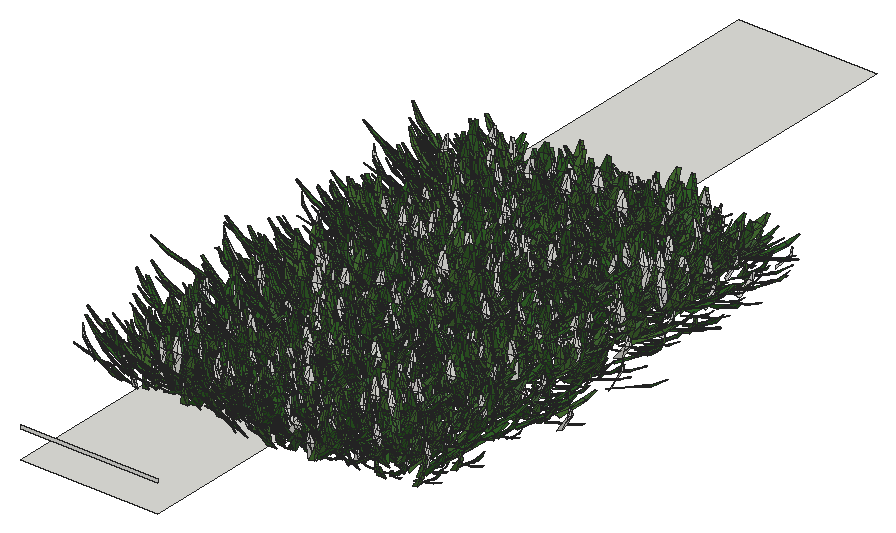
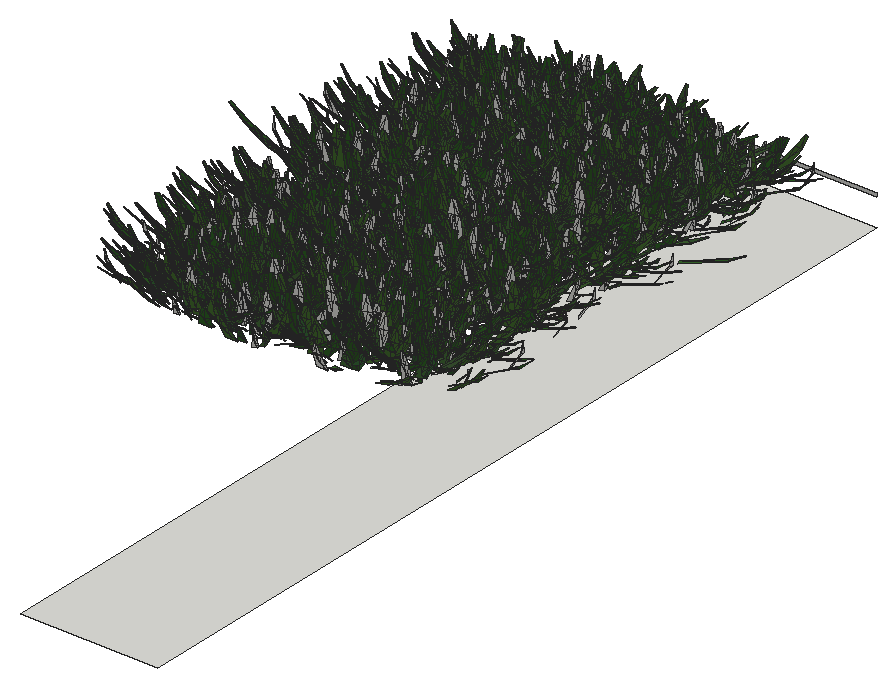
# SketchUp Ruby script. Lengths in inches.
U = 1.inch
M = Sketchup.active_model
def pt(a) = Geom::Point3d.new(a.map { |v| v * U })
def face(e, loops, mat)
  f = e.add_face(loops[0].map { |a| pt(a) })
  loops[1..].each { |l| e.add_face(l.map { |a| pt(a) }).erase! }
  f.material = f.back_material = mat if mat
  f
end
# faces: each face lists its corners as indices into pts; further lists are holes
def faces(e, pts, list, mat = nil) = list.each { |f| face(e, (f[0].is_a?(Array) ? f : [f]).map { |l| l.map { |i| pts[i] } }, mat) }
# xy, xz, yz: faces in a plane at the given z, y or x. An outline is a flat list of corners, or four numbers for a rectangle; further outlines are holes
def ring(l) = l.size == 4 ? [[l[0], l[1]], [l[2], l[1]], [l[2], l[3]], [l[0], l[3]]] : l.each_slice(2).to_a
def flat(e, list, mat, &to3) = list.each { |f| face(e, (f[0].is_a?(Array) ? f : [f]).map { |l| ring(l).map { |u, v| to3.(u, v) } }, mat) }
def xy(e, z, list, mat = nil) = flat(e, list, mat) { |x, y| [x, y, z] }
def xz(e, y, list, mat = nil) = flat(e, list, mat) { |x, z| [x, y, z] }
def yz(e, x, list, mat = nil) = flat(e, list, mat) { |y, z| [x, y, z] }
def lines(e, pts, list) = list.each { |a, b| e.add_line(pt(pts[a]), pt(pts[b])) }
# prism: a flat outline (further loops are holes) pulled along v
def prism(e, loops, v, mat = nil)
  f = face(e, loops, mat); d = Geom::Vector3d.new(v.map { |x| x * U })
  f.pushpull(f.normal.samedirection?(d) ? d.length : -d.length)
end
def box(e, o, s, mat = nil) = prism(e, [[o, [o[0] + s[0], o[1], o[2]], [o[0] + s[0], o[1] + s[1], o[2]], [o[0], o[1] + s[1], o[2]]]], [0, 0, s[2]], mat)
def at(x, y, z, deg = 0) = Geom::Transformation.translation(pt([x, y, z])) * Geom::Transformation.rotation(ORIGIN, Z_AXIS, deg.degrees)
def axes(o, x, y, z) = Geom::Transformation.new([*x, 0, *y, 0, *z, 0, *pt(o).to_a, 1])
def part(name) = M.definitions.add(name)
# library, detail: a bought-in or finely detailed component or shape, given as its bounding box
def library(name, o, s) = part(name).tap { |d| box(d.entities, o, s) }
def detail(e, o, s) = box(e.add_group.entities, o, s)
def put(e, d, t, mat = nil) = e.add_instance(d, t).tap { |i| i.material = mat if mat }
def group(e, t, mat = nil) = e.add_group.tap { |g| g.transformation = t; g.material = mat if mat }.entities
root = M.entities
M.materials.add("Material82").color = [68, 110, 58]
M.materials.add("Material83").color = [48, 90, 38]
M.materials.add("Material84").color = [68, 110, 48]
M.materials.add("Material85").color = [48, 90, 48]
M.materials.add("Material86").color = [58, 110, 58]
M.materials.add("Material87").color = [58, 90, 38]
M.materials.add("Material88").color = [68, 100, 58]
M.materials.add("Material89").color = [48, 100, 38]
c1 = part("grass00")
p = [[-0.6875,0.15,0],[-0.56,0.08,5.52],[-0.04,0.03,2.76],[0.48,-0.02,0],[0.35,-0.02,5.52],[-0.1,-0.14,5.52],
  [-0.12,0.65,8.37],[-0.42,0.65,8.37]]
faces(c1.entities,p,[[0,1,2,3],[3,2,4],[1,5,2],[5,4,2],[1,6,5],[4,5,6],[7,6,1]])
c2 = part("Group16\#1")
put(c2.entities,c1,axes([1.44,-0.61,-0.01],[0.05352,0.12609,0],[-0.10704,0.04543,0.07239],[0.06664,-0.02828,0.11628]),"Material85")
put(c2.entities,c1,axes([0.76,-0.15,-0.01],[0.04676,0.24062,0],[-0.23162,0.04501,0.06642],[0.0652,-0.01267,0.23595]),"Material82")
put(c2.entities,c1,axes([0.79,0.01,-0.01],[-0.00606,0.34651,0],[-0.34381,-0.00602,0.0432],[0.04319,0.00076,0.34386]))
put(c2.entities,c1,axes([1,0.23,-0.01],[-0.07192,0.31144,0],[-0.28722,-0.06632,0.1236],[0.12043,0.02781,0.29478]),"Material84")
put(c2.entities,c1,axes([1.66,0.77,-0.01],[-0.13828,0.29651,0],[-0.21551,-0.1005,0.22471],[0.20365,0.09498,0.23779]),"Material89")
put(c2.entities,c1,axes([0.6875,0.52,-0.01],[-0.18126,0.24051,0],[-0.22746,-0.17142,0.09788],[0.07817,0.05891,0.28481]),"Material84")
put(c2.entities,c1,axes([0.68,0.78,-0.01],[-0.215,0.18688,0],[-0.12385,-0.14248,0.21334],[0.13995,0.16101,0.18878]),"Material82")
put(c2.entities,c1,axes([0.56,1,-0.01],[-0.13756,0.07624,0],[-0.06159,-0.11112,0.0927],[0.04494,0.08108,0.12705]),"Material84")
put(c2.entities,c1,axes([0.2,0.64,-0.01],[-0.23729,0.07254,0],[-0.05711,-0.18681,0.153],[0.04473,0.14632,0.19535]),"Material89")
put(c2.entities,c1,axes([0.0625,0.72,-0.01],[-0.28874,0.02525,0],[-0.02179,-0.24916,0.14647],[0.01276,0.14591,0.25012]),"Material82")
put(c2.entities,c1,axes([-0.08,0.62,-0.01],[-0.34089,-0.04187,0],[0.03255,-0.26504,0.216],[-0.02633,0.21439,0.26703]),"Material89")
put(c2.entities,c1,axes([-0.34,0.98,-0.01],[-0.14314,-0.0493,0],[0.04397,-0.12769,0.06843],[-0.02228,0.0647,0.13505]),"Material89")
put(c2.entities,c1,axes([-0.87,1.45,-0.01],[-0.23488,-0.14114,0],[0.13761,-0.22901,0.06087],[-0.03135,0.05217,0.26717]))
put(c2.entities,c1,axes([-0.72,0.77,-0.01],[-0.14208,-0.13251,0],[0.07209,-0.0773,0.16301],[-0.11118,0.11922,0.1057]),"Material89")
put(c2.entities,c1,axes([-0.62,0.43,-0.01],[-0.14845,-0.21203,0],[0.18654,-0.13061,0.12304],[-0.10079,0.07057,0.22772]),"Material82")
put(c2.entities,c1,axes([-0.68,0.29,-0.01],[-0.13639,-0.32136,0],[0.31723,-0.13464,0.05579],[-0.05136,0.0218,0.34462]),"Material83")
put(c2.entities,c1,axes([-0.64,0.125,-0.01],[-0.0458,-0.23569,0],[0.22124,-0.043,0.08276],[-0.08124,0.01579,0.22538]),"Material86")
put(c2.entities,c1,axes([-1.6,-0.03,-0.01],[0.00576,-0.32897,0],[0.27526,0.00482,0.18018],[-0.18015,-0.00315,0.2753]),"Material84")
put(c2.entities,c1,axes([-1.36,-0.31,-0.01],[0.05718,-0.24765,0],[0.18172,0.04196,0.17267],[-0.16825,-0.03885,0.1865]),"Material89")
put(c2.entities,c1,axes([-1.54,-0.72,-0.01],[0.06537,-0.14017,0],[0.13555,0.06321,0.03939],[-0.0357,-0.01665,0.14956]))
put(c2.entities,c1,axes([-1.19,-0.9,-0.01],[0.09597,-0.12735,0],[0.11214,0.08451,0.07557],[-0.06035,-0.04548,0.14042]),"Material88")
put(c2.entities,c1,axes([-0.47,-0.54,-0.01],[0.11588,-0.10072,0],[0.0618,0.0711,0.12124],[-0.07953,-0.0915,0.0942]))
put(c2.entities,c1,axes([-0.47,-0.84,-0.01],[0.11927,-0.0661,0],[0.06603,0.11913,0.00646],[-0.00313,-0.00565,0.13621]),"Material84")
put(c2.entities,c1,axes([-0.38,-1.24,-0.01],[0.28037,-0.08571,0],[0.0618,0.20215,0.20315],[-0.05939,-0.19428,0.21139]),"Material88")
put(c2.entities,c1,axes([-0.06,-0.66,-0.01],[0.22719,-0.01987,0],[0.01247,0.14255,0.17758],[-0.01547,-0.17691,0.1431]),"Material87")
put(c2.entities,c1,axes([0.11,-0.89,-0.01],[0.14882,0.01828,0],[-0.01058,0.08611,0.12229],[0.01491,-0.12138,0.08676]),"Material85")
put(c2.entities,c1,axes([0.25,-0.72,-0.01],[0.20481,0.07053,0],[-0.06206,0.18022,0.10291],[0.03351,-0.0973,0.1906]),"Material85")
put(c2.entities,c1,axes([0.85,-1.42,-0.01],[0.16481,0.09904,0],[-0.09472,0.15762,0.05616],[0.02893,-0.04814,0.18389]),"Material84")
put(c2.entities,c1,axes([1.01,-1.09,-0.01],[0.21858,0.20385,0],[-0.17495,0.1876,0.15339],[0.10462,-0.11218,0.25652]),"Material89")
put(c2.entities,c1,axes([1.01,-0.71,-0.01],[0.08733,0.12473,0],[-0.06445,0.04512,0.13037],[0.1068,-0.07477,0.07867]),"Material85")
c3 = part("Group15\#1")
put(c3.entities,c2,at(0,0,0))
c4 = part("3darcstudiotree_grass00\#1")
put(c4.entities,c3,at(0,0,0))
xy(root,-42.1875,[[1657.41,273.41,1674.99,387.84]])
xz(root,273.41,[[1657.41,-38.61,1674.99,-38.1875]])
put(root,c4,axes([1666.34,286.12,-34.17],[1.73893,-1.7168,0],[3.5493,0.55914,-0.05078],[0.28442,0.04481,1.72798]))
put(root,c4,axes([1665.54,283.25,-34.17],[1.27117,1.29221,0],[-3.51403,0.53763,-0.02781],[-0.14445,0.0221,1.57422]))
put(root,c4,axes([1667.02,309.98,-34.17],[1.49045,-1.29572,0],[4.01852,0.71892,-0.00454],[0.01627,0.00291,1.30224]))
put(root,c4,axes([1665.8,293.86,-34.17],[3.40006,0.04588,0],[-0.15479,1.78412,-0.02332],[-0.00425,0.049,1.80921]))
put(root,c4,axes([1665.56,329.67,-34.17],[1.48796,1.33204,0],[-3.50735,0.60935,-0.02705],[-0.13278,0.02307,1.54111]))
put(root,c4,axes([1667.26,332.66,-34.17],[-3.4737,0.48099,0],[-1.22806,-1.37939,-0.01418],[-0.03068,-0.03446,1.8149]))
put(root,c4,axes([1666.03,322.07,-34.17],[1.0762,1.29593,0],[-3.71861,0.48029,-0.00037],[-0.00166,0.00021,1.37352]))
put(root,c4,axes([1667.74,303,-34.17],[-4.57816,0.34958,0],[-0.88534,-1.8033,-0.01839],[-0.0151,-0.03075,1.50803]))
put(root,c4,axes([1667.97,291.15,-34.17],[-1.62742,-1.17488,0],[3.69115,-0.79521,-0.05959],[0.21649,-0.04664,1.30502]))
put(root,c4,axes([1667.19,320.27,-34.17],[1.77469,-1.16148,0],[2.86416,0.68064,-0.04784],[0.28474,0.06767,1.7418]))
put(root,c4,axes([1668.11,326.4375,-34.17],[-0.38907,-1.30448,0],[3.64191,-0.16894,-0.01277],[0.06378,-0.00296,1.38207]))
put(root,c4,axes([1666.65,318.48,-34.17],[0.22262,1.70783,0],[-4.21483,0.08545,-0.0387],[-0.20922,0.00424,1.71236]))
put(root,c4,axes([1666.48,306.94,-34.17],[1.40686,1.47706,0],[-4.38712,0.6499,-0.05425],[-0.24934,0.03694,1.72469]))
put(root,c4,axes([1666.91,335.93,-34.17],[3.74197,-0.40965,0],[1.02528,1.45661,-0.05393],[0.09104,0.12934,1.81331]))
put(root,c4,axes([1667.43,289.47,-34.17],[-1.63246,1.63511,0],[-3.4831,-0.54085,-0.00571],[-0.03452,-0.00536,1.8245]))
put(root,c4,axes([1667.63,298.92,-34.17],[-0.95146,1.7451,0],[-3.70497,-0.31417,-0.03186],[-0.21482,-0.01822,1.95913]))
put(root,c4,axes([1668.68,331.43,-34.17],[3.26505,-0.4107,0],[1.3901,1.71877,-0.05774],[0.0978,0.12093,1.91123]))
put(root,c4,axes([1668.51,314.42,-34.17],[2.80643,0.90661,0],[-2.10951,1.0156,-0.00694],[-0.02809,0.01352,1.5947]))
put(root,c4,axes([1668.74,296.95,-34.17],[4.57178,0.1006,0],[-0.19659,1.38952,-0.03032],[-0.00983,0.06951,1.54015]))
put(root,c4,axes([1670.42,331.34,-34.17],[-3.18088,-0.40858,0],[1.35408,-1.63957,-0.00123],[0.00227,-0.00275,1.95221]))
put(root,c4,axes([1671.25,296.25,-34.17],[-2.17426,-1.31341,0],[3.93463,-1.01304,-0.04707],[0.15585,-0.04013,1.39282]))
put(root,c4,axes([1670.89,287.45,-34.17],[-3.35474,0.10257,0],[-0.29043,-1.4774,-0.03359],[-0.01806,-0.09187,1.95875]))
put(root,c4,axes([1670.53,318.16,-34.17],[3.26089,-0.9276,0],[2.41726,1.32164,-0.00659],[0.02436,0.01332,1.95827]))
put(root,c4,axes([1670.33,283.82,-34.17],[3.92346,-0.38379,0],[1.02863,1.63546,-0.04456],[0.04806,0.07641,1.43455]))
put(root,c4,axes([1672,313.41,-34.17],[-3.24318,-0.61658,0],[1.47082,-1.20323,-0.00927],[0.0316,-0.02585,1.99366]))
put(root,c4,axes([1672.55,293.77,-34.17],[-0.91872,-1.28532,0],[4.49567,-0.49978,-0.01485],[0.07367,-0.00819,1.80381]))
put(root,c4,axes([1671.83,307.1,-34.17],[0.6017,-1.37989,0],[3.88457,0.26344,-0.05034],[0.29768,0.02019,1.77282]))
put(root,c4,axes([1671.1875,285.4,-34.17],[3.93415,-0.89756,0],[1.9948,1.35987,-0.042],[0.11006,0.07503,1.56273]))
put(root,c4,axes([1671.37,335.04,-34.17],[-1.11116,1.30676,0],[-3.31516,-0.43843,-0.03292],[-0.23061,-0.0305,1.93659]))
put(root,c4,axes([1672.71,319.98,-34.17],[-1.52685,-1.32373,0],[3.20025,-0.57411,-0.03768],[0.23061,-0.04137,1.77164]))
put(root,c4,axes([1671.8,325.38,-34.17],[-1.03634,1.43503,0],[-4.07668,-0.45789,-0.05457],[-0.22787,-0.02559,1.37935]))
put(root,c4,axes([1673.05,326.875,-34.17],[-3.57412,-0.0033,0],[0.00935,-1.57631,-0.04252],[0.00057,-0.09613,1.71753]))
put(root,c4,axes([1672.76,323.15,-34.17],[1.46562,-1.72266,0],[4.03529,0.53396,-0.04434],[0.25483,0.03372,1.93394]))
put(root,c4,axes([1671.59,304.17,-34.17],[3.29517,0.70525,0],[-2.24642,1.63243,-0.00178],[-0.00323,0.00235,1.34491]))
put(root,c4,axes([1673.5,291.3,-34.17],[-3.95181,0.01249,0],[-0.03447,-1.69649,-0.00779],[-0.00033,-0.01629,1.71052]))
put(root,c4,axes([1672.0625,332.5625,-34.17],[0.85595,1.34318,0],[-4.39323,0.43542,-0.04255],[-0.19043,0.01887,1.5668]))
put(root,c4,axes([1673.12,298.65,-34.17],[2.65299,-0.97546,0],[3.20943,1.35758,-0.02398],[0.06395,0.02705,1.37951]))
put(root,c4,axes([1672.28,315.24,-34.17],[-0.08871,1.46443,0],[-4.0853,-0.03849,-0.0357],[-0.16722,-0.00158,1.43525]))
put(root,c4,axes([1672.9375,302.09,-34.17],[-1.54224,1.54277,0],[-3.96225,-0.61604,-0.03242],[-0.18554,-0.02885,1.96368]))
put(root,c4,axes([1673.8,289.625,-34.17],[1.45525,-1.36358,0],[3.3603,0.55776,-0.00467],[0.02235,0.00371,1.41828]))
put(root,c4,axes([1673.26,328.28,-34.17],[3.00061,-1.20381,0],[2.59687,1.00673,-0.02297],[0.10061,0.039,1.67632]))
put(root,c4,axes([1673.2,338.31,-34.17],[3.81318,-1.10593,0],[2.582,1.38461,-0.02397],[0.05758,0.03088,1.32443]))
put(root,c4,axes([1674.27,300.13,-34.17],[-4.06047,-0.30244,0],[0.85134,-1.77769,-0.03943],[0.03436,-0.07175,1.61444]))
put(root,c4,axes([1672.76,311.82,-34.17],[4.70379,-0.18713,0],[0.44198,1.72795,-0.01121],[0.00446,0.01743,1.30781]))
put(root,c4,axes([1673.62,309.8,-34.17],[4.53982,0.21063,0],[-0.49544,1.66085,-0.02625],[-0.01899,0.06364,1.96735]))
put(root,c4,axes([1675.79,287.28,-34.17],[-3.49662,-0.83415,0],[2.45665,-1.60161,-0.00291],[0.00652,-0.00425,1.54121]))
put(root,c4,axes([1675.96,296.14,-34.17],[0.98995,-1.43102,0],[4.03348,0.43397,-0.01691],[0.08344,0.00898,1.6028]))
put(root,c4,axes([1676.05,319.87,-34.17],[2.00913,-1.08398,0],[3.65765,1.05439,-0.0361],[0.15471,0.0446,1.80295]))
put(root,c4,axes([1675.89,333.45,-34.17],[-2.26736,0.9467,0],[-3.26135,-1.21483,-0.01576],[-0.0639,-0.0238,1.87507]))
put(root,c4,axes([1676.31,310.1,-34.17],[3.78243,-0.20016,0],[0.50434,1.48226,-0.04419],[0.03105,0.09126,1.50171]))
put(root,c4,axes([1677.36,330.47,-34.17],[-3.45253,0.27622,0],[-0.72182,-1.40321,-0.01756],[-0.02267,-0.04407,1.76676]))
put(root,c4,axes([1676.19,283.46,-34.17],[3.16343,0.45899,0],[-1.51538,1.62437,-0.05896],[-0.12026,0.12891,1.94308]))
put(root,c4,axes([1677.36,335.34,-34.17],[0.78455,-1.57227,0],[3.87046,0.30038,-0.05061],[0.32766,0.02543,1.95081]))
put(root,c4,axes([1677.9,314.09,-34.17],[-4.25587,0.04591,0],[-0.1089,-1.57017,-0.04984],[-0.00682,-0.0984,1.49526]))
put(root,c4,axes([1677.88,315.32,-34.17],[0.66389,-1.49509,0],[4.57403,0.31589,-0.04237],[0.23153,0.01599,1.93074]))
put(root,c4,axes([1677.33,307.87,-34.17],[-2.17136,1.02025,0],[-2.89421,-0.95801,-0.02769],[-0.1122,-0.03714,1.49833]))
put(root,c4,axes([1677.42,300.01,-34.17],[-1.21684,1.60263,0],[-3.24686,-0.38342,-0.04102],[-0.25836,-0.03051,1.67021]))
put(root,c4,axes([1677.96,298.69,-34.17],[-3.24632,0.41503,0],[-1.13877,-1.38534,-0.02033],[-0.04358,-0.05301,1.92362]))
put(root,c4,axes([1677.0625,326.37,-34.17],[3.77678,0.27869,0],[-0.6902,1.45473,-0.00485],[-0.00557,0.01174,1.75633]))
put(root,c4,axes([1676.94,289.48,-34.17],[0.70399,1.48206,0],[-4.34932,0.32132,-0.00799],[-0.0357,0.00264,1.50733]))
put(root,c4,axes([1677.66,303.2,-34.17],[4.36912,-0.54802,0],[1.07763,1.33621,-0.00335],[0.00554,0.00687,1.45436]))
put(root,c4,axes([1678.55,337.63,-34.17],[1.61856,-1.20753,0],[3.98562,0.83088,-0.05061],[0.25894,0.05398,1.95538]))
put(root,c4,axes([1679.33,284.88,-34.17],[-4.39724,-0.41789,0],[0.97106,-1.58919,-0.03666],[0.03598,-0.05889,1.30149]))
put(root,c4,axes([1679.63,291.59,-34.17],[-3.07103,-1.30718,0],[3.25603,-1.18973,-0.02123],[0.06738,-0.02462,1.43939]))
put(root,c4,axes([1678.17,318.12,-34.17],[3.97153,-0.13343,0],[0.30373,1.40602,-0.01096],[0.00672,0.03109,1.93666]))
put(root,c4,axes([1679.47,324.36,-34.17],[0.94741,-1.42267,0],[3.73003,0.38633,-0.03356],[0.18091,0.01874,1.61101]))
put(root,c4,axes([1678.45,294.03,-34.17],[3.9873,-0.15062,0],[0.35569,1.46445,-0.02913],[0.01977,0.08141,1.9903]))
put(root,c4,axes([1679.81,311.43,-34.17],[0.11291,-1.83708,0],[4.52912,0.0433,-0.04883],[0.22915,0.00219,1.59403]))
put(root,c4,axes([1678.15,304.79,-34.17],[1.39223,1.25256,0],[-3.795,0.65605,-0.01361],[-0.06427,0.01111,1.60179]))
put(root,c4,axes([1678.93,322.18,-34.17],[4.35154,-0.63119,0],[1.42423,1.52711,-0.01984],[0.04228,0.04533,1.90869]))
put(root,c4,axes([1679.34,328.61,-34.17],[2.81234,1.34734,0],[-2.81254,0.91306,-0.01155],[-0.05543,0.018,1.69697]))
put(root,c4,axes([1681.53,301.41,-34.17],[-3.18803,-0.40221,0],[1.38309,-1.70502,-0.00535],[0.00805,-0.00992,1.67969]))
put(root,c4,axes([1681.68,309.92,-34.17],[0.12157,-1.62148,0],[4.39568,0.05126,-0.0158],[0.08264,0.00096,1.72451]))
put(root,c4,axes([1681.9375,289.96,-34.17],[0.05707,-1.33182,0],[4.67038,0.03113,-0.02351],[0.10833,0.00072,1.61343]))
put(root,c4,axes([1681.33,297.8125,-34.17],[2.55829,-1.10547,0],[3.21956,1.15881,-0.03913],[0.13719,0.04938,1.55084]))
put(root,c4,axes([1682.01,315.66,-34.17],[-4.65824,0.34825,0],[-0.74927,-1.55877,-0.04366],[-0.04609,-0.09588,1.70895]))
put(root,c4,axes([1682.33,307.59,-34.17],[-4.52964,-0.09494,0],[0.22898,-1.69903,-0.02618],[0.00745,-0.05528,1.73378]))
put(root,c4,axes([1682.67,326.74,-34.17],[-3.60203,-0.72226,0],[1.64221,-1.27378,-0.05096],[0.13667,-0.10601,1.60728]))
put(root,c4,axes([1681.43,325.2,-34.17],[3.44825,-0.26897,0],[0.66516,1.32629,-0.00259],[0.00332,0.00662,1.70099]))
put(root,c4,axes([1681.76,320.69,-34.17],[3.35413,-0.63199,0],[1.61191,1.33051,-0.01719],[0.04506,0.03719,1.70421]))
put(root,c4,axes([1683.05,331.67,-34.17],[-3.59651,-0.44623,0],[1.25179,-1.56915,-0.00258],[0.00335,-0.0042,1.35273]))
put(root,c4,axes([1683.37,291.83,-34.17],[-3.14814,-1.33954,0],[3.08708,-1.12839,-0.01903],[0.08494,-0.03105,1.91973]))
put(root,c4,axes([1682.36,302.16,-34.17],[-2.16052,1.42464,0],[-3.02099,-0.71254,-0.01081],[-0.04852,-0.01144,1.38013]))
put(root,c4,axes([1682.83,335.55,-34.17],[1.98347,-1.087,0],[3.74124,1.06175,-0.05142],[0.23843,0.06767,1.97373]))
put(root,c4,axes([1681.92,305.125,-34.17],[1.97793,1.10174,0],[-3.47293,0.96971,-0.06047],[-0.20758,0.05796,1.34144]))
put(root,c4,axes([1683.66,329.35,-34.17],[-1.19412,-1.34448,0],[3.1862,-0.44013,-0.02961],[0.14836,-0.02049,1.34337]))
put(root,c4,axes([1682.78,296.48,-34.17],[-1.72626,1.58438,0],[-3.31687,-0.56206,-0.02574],[-0.1159,-0.01964,1.32606]))
put(root,c4,axes([1682.78,314.18,-34.17],[2.97087,-0.63768,0],[1.76888,1.28171,-0.04084],[0.13668,0.09904,1.94165]))
put(root,c4,axes([1684.41,318.24,-34.17],[-2.73035,-0.81396,0],[2.55013,-1.33042,-0.03674],[0.11326,-0.05909,1.62045]))
put(root,c4,axes([1684.4,286.92,-34.17],[-4.52935,0.02332,0],[-0.05756,-1.73901,-0.02897],[-0.00164,-0.04958,1.4344]))
put(root,c4,axes([1683.26,332.6875,-34.17],[3.47707,-0.28838,0],[0.88445,1.65855,-0.04208],[0.03591,0.06734,1.3356]))
put(root,c4,axes([1683.17,283.95,-34.17],[3.17869,1.06939,0],[-2.97014,1.37309,-0.05603],[-0.1904,0.08802,1.79617]))
put(root,c4,axes([1684.53,294.24,-34.17],[-2.94959,0.77761,0],[-1.85667,-1.09533,-0.00767],[-0.02785,-0.01643,1.63569]))
put(root,c4,axes([1684.83,323.12,-34.17],[1.55533,-1.52655,0],[4.26431,0.67573,-0.03894],[0.20513,0.0325,1.95573]))
put(root,c4,axes([1684.68,312.12,-34.17],[2.20471,-1.56419,0],[3.09714,0.67895,-0.02727],[0.12975,0.02844,1.44583]))
put(root,c4,axes([1685.1,339.89,-34.17],[0.44293,-1.56057,0],[3.90028,0.17217,-0.04376],[0.2246,0.00991,1.51939]))
put(root,c4,axes([1684.13,285.08,-34.17],[4.17705,-0.03481,0],[0.09875,1.84286,-0.00824],[0.00079,0.01483,1.59977]))
put(root,c4,axes([1684.7,337.99,-34.17],[-2.26608,1.33318,0],[-3.11704,-0.82402,-0.02214],[-0.10686,-0.02825,1.63462]))
put(root,c4,axes([1684.54,281.59,-34.17],[3.74746,0.48768,0],[-1.05117,1.25627,-0.0401],[-0.08448,0.10096,1.69032]))
put(root,c4,axes([1686.92,318.45,-34.17],[-4.55367,0.27818,0],[-0.67765,-1.72528,-0.03016],[-0.02264,-0.05764,1.62739]))
put(root,c4,axes([1687.875,305.5625,-34.17],[-1.63823,-1.36099,0],[3.49292,-0.65391,-0.00409],[0.01763,-0.0033,1.3842]))
put(root,c4,axes([1687.32,282.83,-34.17],[-3.4101,0.33219,0],[-0.86784,-1.38556,-0.03348],[-0.045,-0.07185,1.52035]))
put(root,c4,axes([1687.74,306.59,-34.17],[2.36777,-1.25491,0],[3.70344,1.08678,-0.00846],[0.02737,0.00803,1.39582]))
put(root,c4,axes([1688.55,330.67,-34.17],[-4.42879,-0.33071,0],[0.76141,-1.58586,-0.02653],[0.02727,-0.05679,1.69452]))
put(root,c4,axes([1688.54,299,-34.17],[-3.60435,-0.22712,0],[0.60496,-1.49319,-0.01241],[0.00897,-0.02215,1.31731]))
put(root,c4,axes([1687.44,311.36,-34.17],[3.96894,-0.58875,0],[1.33194,1.3965,-0.01237],[0.02838,0.02976,1.84855]))
put(root,c4,axes([1688.94,286.82,-34.17],[-3.95806,-0.26007,0],[0.56997,-1.34913,-0.01531],[0.01744,-0.04128,1.80136]))
put(root,c4,axes([1688.8,291.09,-34.17],[0.93986,-1.61608,0],[3.43783,0.31095,-0.013],[0.09422,0.00852,1.96601]))
put(root,c4,axes([1689.21,294.27,-34.17],[-0.9687,-1.6973,0],[3.99206,-0.35436,-0.03143],[0.1527,-0.01355,1.52743]))
put(root,c4,axes([1689.51,316.53,-34.17],[-1.5733,-1.53629,0],[3.8056,-0.60614,-0.01424],[0.06159,-0.00981,1.43479]))
put(root,c4,axes([1689.37,332.76,-34.17],[-3.45853,-0.30921,0],[0.875,-1.52216,-0.03754],[0.05438,-0.09459,1.94323]))
put(root,c4,axes([1689.07,295.6,-34.17],[-0.43954,-1.59759,0],[3.53501,-0.15126,-0.05057],[0.33495,-0.01433,1.77563]))
put(root,c4,axes([1688.06,309.33,-34.17],[3.08639,0.66231,0],[-1.76537,1.27948,-0.04213],[-0.09869,0.07153,1.35679]))
put(root,c4,axes([1689.27,290.28,-34.17],[2.93587,-1.18133,0],[2.75704,1.06566,-0.0131],[0.05816,0.02248,1.79861]))
put(root,c4,axes([1690.12,319.46,-34.17],[-3.47148,-0.32447,0],[1.09042,-1.81447,-0.00987],[0.00954,-0.01587,1.48448]))
put(root,c4,axes([1688.3,302.78,-34.17],[3.59479,1.11581,0],[-2.65109,1.32837,-0.01986],[-0.0739,0.03703,1.93312]))
put(root,c4,axes([1689.12,285.5625,-34.17],[-0.72391,1.71321,0],[-3.27988,-0.21555,-0.00349],[-0.01869,-0.00123,1.35435]))
put(root,c4,axes([1689.125,337.3125,-34.17],[3.93037,0.00712,0],[-0.01552,1.3324,-0.03904],[-0.00131,0.11261,1.85207]))
put(root,c4,axes([1690.13,299.85,-34.17],[1.97331,-1.7001,0],[3.41411,0.61633,-0.04178],[0.21918,0.03957,1.62381]))
put(root,c4,axes([1689.27,313.02,-34.17],[3.30561,0.92504,0],[-2.54174,1.41264,-0.05586],[-0.15004,0.08339,1.52805]))
put(root,c4,axes([1690.21,329.125,-34.17],[3.0975,-0.44176,0],[1.39811,1.52468,-0.04794],[0.07202,0.07854,1.36124]))
put(root,c4,axes([1690.95,327.59,-34.17],[2.99585,-0.78884,0],[2.43675,1.4393,-0.03164],[0.10153,0.05997,1.90074]))
put(root,c4,axes([1690.59,335.03,-34.17],[4.2542,-0.55295,0],[1.2277,1.46904,-0.0158],[0.03318,0.0397,1.97161]))
put(root,c4,axes([1690.24,325.14,-34.17],[1.7248,1.72946,0],[-3.94677,0.61218,-0.01805],[-0.10059,0.0156,1.90362]))
put(root,c4,axes([1690.24,339.14,-34.17],[0.74688,1.42324,0],[-4.33801,0.35406,-0.00233],[-0.01216,0.00099,1.77271]))
put(root,c4,axes([1690.79,321.9375,-34.17],[4.44722,-0.53115,0],[1.26492,1.64719,-0.03542],[0.04521,0.05887,1.44036]))
put(root,c4,axes([1692.55,305.17,-34.17],[-2.92804,-0.86099,0],[2.52273,-1.33432,-0.01853],[0.05328,-0.02818,1.52144]))
put(root,c4,axes([1692.84,316.7,-34.17],[-3.6982,-1.11774,0],[2.6803,-1.37926,-0.01589],[0.04062,-0.0209,1.38765]))
put(root,c4,axes([1692.52,322.29,-34.17],[-4.1478,0.13224,0],[-0.279,-1.36104,-0.02584],[-0.01399,-0.06822,1.74304]))
put(root,c4,axes([1692.41,329.11,-34.17],[2.38875,-0.89777,0],[2.38741,0.98797,-0.03437],[0.15253,0.06312,1.66865]))
put(root,c4,axes([1693.1,333.22,-34.17],[0.38467,-1.72776,0],[3.7527,0.12994,-0.02351],[0.1369,0.00474,1.65028]))
put(root,c4,axes([1693.69,339.19,-34.17],[-0.80049,-1.46058,0],[4.26303,-0.36338,-0.06129],[0.24511,-0.02089,1.3376]))
put(root,c4,axes([1692.5,300.5,-34.17],[3.0128,0.96923,0],[-2.26467,1.09486,-0.0073],[-0.03331,0.01611,1.93831]))
put(root,c4,axes([1694.47,334.76,-34.17],[-4.20928,0.13814,0],[-0.29813,-1.41294,-0.01346],[-0.00713,-0.03379,1.72106]))
put(root,c4,axes([1694.72,287.39,-34.17],[-3.15856,-0.38514,0],[1.26271,-1.61061,-0.02785],[0.04659,-0.05943,1.81462]))
put(root,c4,axes([1694.05,292.03,-34.17],[-1.513,1.21159,0],[-3.36011,-0.6526,-0.03193],[-0.17356,-0.03371,1.70102]))
put(root,c4,axes([1695.18,298.42,-34.17],[-3.75328,0.12847,0],[-0.28677,-1.30306,-0.03872],[-0.02406,-0.10934,1.78675]))
put(root,c4,axes([1693.92,337.64,-34.17],[3.29344,0.56908,0],[-1.86687,1.68036,-0.0492],[-0.08744,0.0787,1.54416]))
put(root,c4,axes([1694.23,294.05,-34.17],[3.21716,0.40848,0],[-1.16198,1.42335,-0.048],[-0.09517,0.11657,1.83855]))
put(root,c4,axes([1695.63,331.08,-34.17],[0.99609,-1.23763,0],[4.45512,0.55768,-0.04397],[0.17141,0.02146,1.43296]))
put(root,c4,axes([1696.39,309.81,-34.17],[-1.04498,-1.27032,0],[4.0983,-0.52433,-0.01227],[0.0665,-0.00851,1.83962]))
put(root,c4,axes([1695.95,326.91,-34.17],[1.40396,-1.3283,0],[3.66211,0.60201,-0.02113],[0.09939,0.01634,1.51549]))
put(root,c4,axes([1694.5,318.02,-34.17],[1.27309,1.64144,0],[-4.4392,0.53549,-0.03143],[-0.12353,0.0149,1.42994]))
put(root,c4,axes([1695.23,310.79,-34.17],[3.7109,-0.91214,0],[2.11846,1.34044,-0.04378],[0.13838,0.08756,1.79394]))
put(root,c4,axes([1694.92,313.16,-34.17],[3.34228,0.13265,0],[-0.43082,1.68835,-0.00091],[-0.00041,0.00162,1.45853]))
put(root,c4,axes([1694.82,302.97,-34.17],[0.73987,1.59354,0],[-4.44696,0.32112,-0.04305],[-0.22862,0.01651,1.82947]))
put(root,c4,axes([1694.97,286.08,-34.17],[3.16975,0.46707,0],[-1.43384,1.51339,-0.02415],[-0.05301,0.05595,1.92547]))
put(root,c4,axes([1695.27,306.83,-34.17],[0.58066,1.77085,0],[-3.90665,0.19923,-0.04685],[-0.26361,0.01344,1.67517]))
put(root,c4,axes([1696.46,319.93,-34.17],[1.02841,-1.31305,0],[3.38391,0.41221,-0.03395],[0.18437,0.02246,1.50895]))
put(root,c4,axes([1695.48,283.7,-34.17],[2.81615,0.69239,0],[-1.81737,1.14964,-0.0044],[-0.01183,0.00748,1.30779]))
put(root,c4,axes([1695.49,324.42,-34.17],[3.53019,1.19751,0],[-2.61374,1.19838,-0.04839],[-0.15514,0.07113,1.47711]))
put(root,c4,axes([1695.6,289.2,-34.17],[3.28885,0.70173,0],[-2.10741,1.53616,-0.00222],[-0.00511,0.00372,1.6055]))
put(root,c4,axes([1696.09,296.4,-34.17],[3.3322,0.38036,0],[-1.11394,1.51777,-0.02015],[-0.03056,0.04163,1.63787]))
put(root,c4,axes([1698.57,300.84,-34.17],[-2.43541,-1.16543,0],[2.64027,-0.85812,-0.03867],[0.17422,-0.05662,1.49724]))
